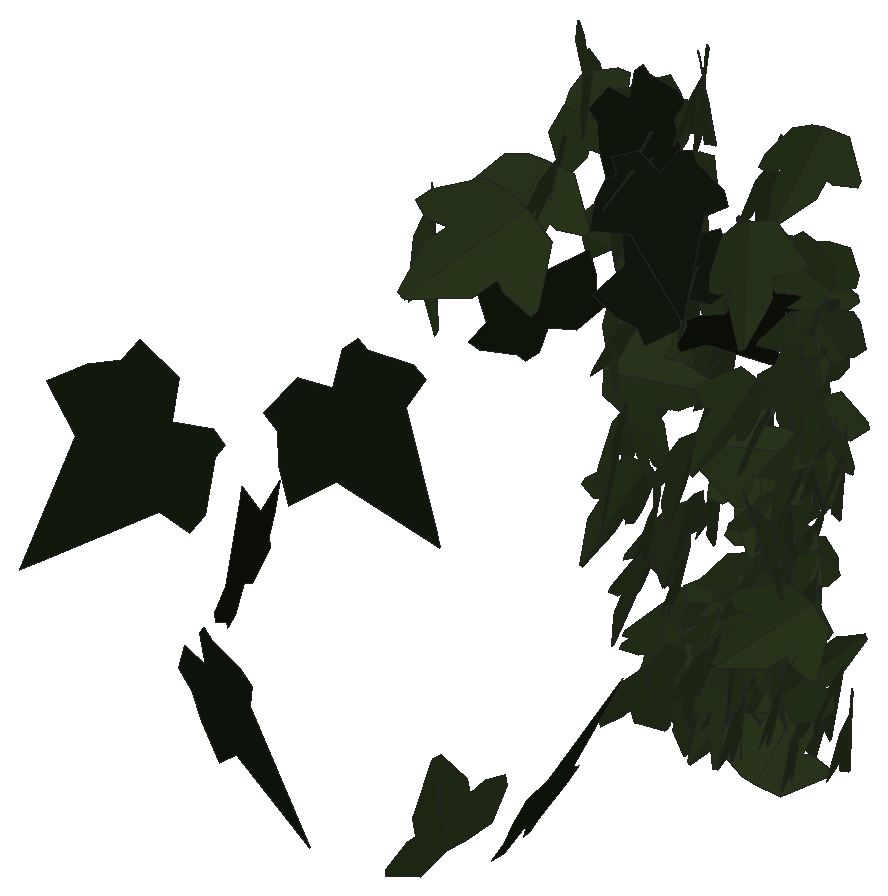
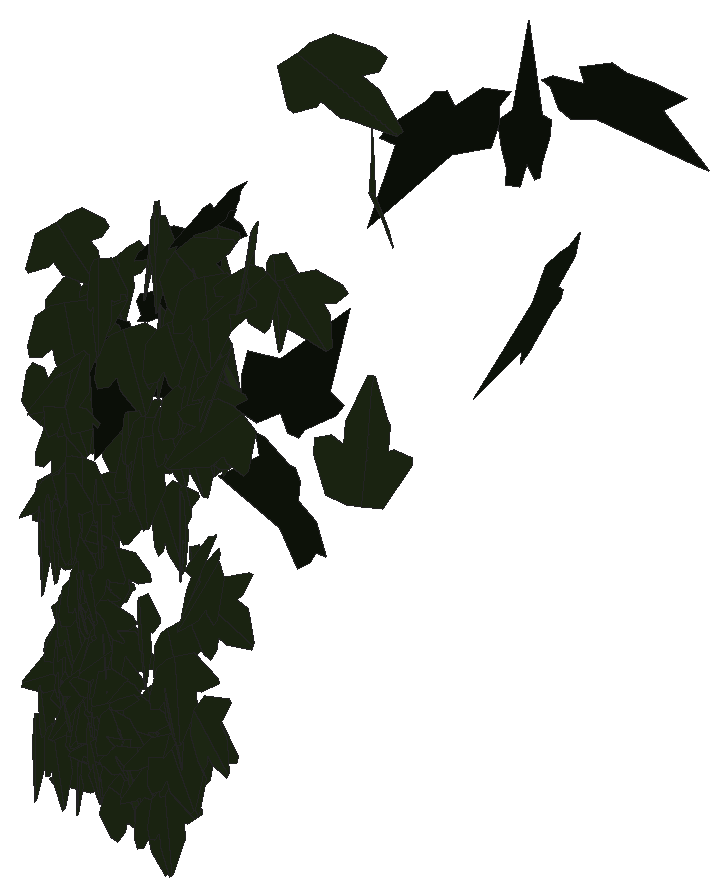
# SketchUp Ruby script. Lengths in inches.
U = 1.inch
M = Sketchup.active_model
def pt(a) = Geom::Point3d.new(a.map { |v| v * U })
def face(e, loops, mat)
  f = e.add_face(loops[0].map { |a| pt(a) })
  loops[1..].each { |l| e.add_face(l.map { |a| pt(a) }).erase! }
  f.material = f.back_material = mat if mat
  f
end
# faces: each face lists its corners as indices into pts; further lists are holes
def faces(e, pts, list, mat = nil) = list.each { |f| face(e, (f[0].is_a?(Array) ? f : [f]).map { |l| l.map { |i| pts[i] } }, mat) }
# xy, xz, yz: faces in a plane at the given z, y or x. An outline is a flat list of corners, or four numbers for a rectangle; further outlines are holes
def ring(l) = l.size == 4 ? [[l[0], l[1]], [l[2], l[1]], [l[2], l[3]], [l[0], l[3]]] : l.each_slice(2).to_a
def flat(e, list, mat, &to3) = list.each { |f| face(e, (f[0].is_a?(Array) ? f : [f]).map { |l| ring(l).map { |u, v| to3.(u, v) } }, mat) }
def xy(e, z, list, mat = nil) = flat(e, list, mat) { |x, y| [x, y, z] }
def xz(e, y, list, mat = nil) = flat(e, list, mat) { |x, z| [x, y, z] }
def yz(e, x, list, mat = nil) = flat(e, list, mat) { |y, z| [x, y, z] }
def lines(e, pts, list) = list.each { |a, b| e.add_line(pt(pts[a]), pt(pts[b])) }
# prism: a flat outline (further loops are holes) pulled along v
def prism(e, loops, v, mat = nil)
  f = face(e, loops, mat); d = Geom::Vector3d.new(v.map { |x| x * U })
  f.pushpull(f.normal.samedirection?(d) ? d.length : -d.length)
end
def box(e, o, s, mat = nil) = prism(e, [[o, [o[0] + s[0], o[1], o[2]], [o[0] + s[0], o[1] + s[1], o[2]], [o[0], o[1] + s[1], o[2]]]], [0, 0, s[2]], mat)
def at(x, y, z, deg = 0) = Geom::Transformation.translation(pt([x, y, z])) * Geom::Transformation.rotation(ORIGIN, Z_AXIS, deg.degrees)
def axes(o, x, y, z) = Geom::Transformation.new([*x, 0, *y, 0, *z, 0, *pt(o).to_a, 1])
def part(name) = M.definitions.add(name)
# library, detail: a bought-in or finely detailed component or shape, given as its bounding box
def library(name, o, s) = part(name).tap { |d| box(d.entities, o, s) }
def detail(e, o, s) = box(e.add_group.entities, o, s)
def put(e, d, t, mat = nil) = e.add_instance(d, t).tap { |i| i.material = mat if mat }
def group(e, t, mat = nil) = e.add_group.tap { |g| g.transformation = t; g.material = mat if mat }.entities
root = M.entities
M.materials.add("efeu1").color = [18, 25, 13]
M.materials.add("efeu2").color = [43, 57, 29]
c1 = part("ivyleaf_10")
p = [[0,0.5,-0.03],[-0.0625,2.02,-0.43],[-0.19,2.01,-0.46],[-0.54,1.05,-0.29],[-0.52,0.625,-0.18],[-0.83,0.76,-0.28],
  [-1.16,0.64,-0.33],[-1.15,0.33,-0.24],[-0.77,-0.39,0.02],[-0.3,-0.51,0.16],[0.04,-0.48,0.23],[-0.02,2.01,-0.4375],
  [-0.06,2.01,-0.43],[0.04,-0.49,0.23],[0.67,-0.49,0.14],[1.38,0.36,-0.2],[1.375,0.51,-0.24],[0.81,0.65,-0.19],
  [0.62,0.59,-0.15],[0.6,1.09,-0.28],[0.5,1.23,-0.31]]
faces(c1.entities,p,[[0,1,2,3,4,5,6,7,8,9,10],[11,12,0,13,14,15,16,17,18,19,20]],"efeu2")
c2 = part("ivyleaf_9")
p = [[1.54,2.16,1.25],[1.36,2.04,1.19],[-0.21,0.99,0.68],[-0.71,1.11,0.82],[-0.85,0.86,0.67],[-0.8,0.17,0.21],
  [-0.9,-0.01,0.1],[-0.67,-0.16,-0.02],[-0.08,-0.08,-0.05],[-0.03,-0.6,-0.4],[0.65,-0.88,-0.66],[0.83,-0.6,-0.49],
  [1.29,-0.42,-0.43],[1.8125,-0.07,-0.26],[1.21,0.44,0.15]]
faces(c2.entities,p,[[0,1,2,3,4,5,6,7,8,9,10,11,12,13,14]],"efeu1")
put(root,c1,axes([498.77,137.96,174.09],[0.169,-0.58916,0.2344],[0.04707,-0.23026,-0.61268],[0.63233,0.17461,-0.01704]))
put(root,c1,axes([498.98,136.23,183.62],[0.22181,-0.25237,-0.641],[-0.15269,0.63865,-0.30428],[0.67176,0.2285,0.14249]))
put(root,c2,axes([499.04,135.21,179.7],[0.2917,0.13697,0.71958],[-0.66782,-0.2685,0.32182],[0.30096,-0.72856,0.01668]))
put(root,c1,axes([498.87,137.54,177.1],[0.09454,-0.25751,-0.64935],[0.04934,0.6561,-0.253],[0.6968,-0.01152,0.10602]))
put(root,c1,axes([498.57,137.53,180.49],[-0.42749,-0.20493,-0.51144],[0.47103,0.19988,-0.47381],[0.28582,-0.6359,0.01589]))
put(root,c1,axes([498.9375,135.04,182.21],[0.61517,0.37241,-0.28496],[-0.24312,-0.14865,-0.71911],[-0.40097,0.66147,-0.00117]))
put(root,c1,axes([498.82,137.39,181.62],[-0.21092,0.66772,0.08289],[-0.00673,0.08477,-0.69999],[-0.67281,-0.21017,-0.01899]))
put(root,c2,axes([499.37,125.42,182.29],[-1.05986,-0.37028,0.11023],[-0.10675,-0.03827,-1.09083],[0.40203,-0.98631,0.00094]))
put(root,c1,axes([498.85,136.36,182.875],[-0.09912,-0.44323,-0.59194],[0.43722,0.44654,-0.40757],[0.5964,-0.40103,0.20041]))
put(root,c1,axes([499.23,135.13,182.51],[0.14096,-0.64935,-0.25041],[-0.0615,0.24288,-0.66443],[0.69324,0.15358,-0.00802]))
put(root,c1,axes([499.22,137.11,176.09],[-0.01704,-0.53595,0.46997],[0.03181,-0.47021,-0.53507],[0.71211,0.00818,0.03515]))
put(root,c1,axes([499.3125,137.19,182.9],[-0.2777,-0.65594,-0.01572],[0.00632,0.01439,-0.71231],[0.6561,-0.27777,0.00021]))
put(root,c1,axes([499.32,138.36,172.28],[-0.0191,-0.63454,-0.11075],[-0.01416,0.11119,-0.63459],[0.64398,-0.01637,-0.01724]))
put(root,c1,axes([499.33,138.07,175.02],[-0.14804,-0.64309,-0.06517],[0.00793,0.06505,-0.65987],[0.64633,-0.14809,-0.00683]))
put(root,c1,axes([499.4,138.1,173.32],[-0.20336,-0.59074,0.1892],[-0.01618,-0.19399,-0.62308],[0.62009,-0.1988,0.04579]))
put(root,c1,axes([499.42,137.98,173.15],[-0.18925,-0.59193,0.19072],[-0.02305,-0.19254,-0.62046],[0.62147,-0.1874,0.03507]))
put(root,c1,axes([499.36,137.16,177.29],[-0.2726,0.54581,0.3087],[-0.11192,0.28886,-0.60955],[-0.61699,-0.29355,-0.02582]))
put(root,c1,axes([499.55,137.32,180.62],[-0.40426,-0.52725,0.21041],[-0.06228,-0.21556,-0.65981],[0.56426,-0.40154,0.07793]))
put(root,c1,axes([499.48,138.05,174.4],[0.29468,-0.58013,-0.09412],[-0.02556,0.09253,-0.6504],[0.58716,0.29518,0.01892]))
put(root,c1,axes([499.55,137.61,178.39],[0.35782,-0.54445,-0.20408],[0.01661,0.2491,-0.63544],[0.5812,0.32808,0.1438]))
put(root,c1,axes([499.62,138.35,172.09],[-0.0688,-0.63941,0.05428],[-0.00276,-0.05429,-0.64309],[0.6417,-0.06879,0.00305]))
put(root,c1,axes([499.53,137.12,181.4],[0.06691,-0.6186,-0.31639],[0.11539,0.32334,-0.60777],[0.68517,0.00596,0.13325]))
put(root,c1,axes([499.49,138.25,173.5],[0.10922,0.6266,0.06189],[-0.00272,0.06328,-0.6359],[-0.62964,0.10842,0.01348]))
put(root,c1,axes([499.68,137.76,175.4],[-0.01368,-0.66531,0.04219],[0.00323,-0.04226,-0.66543],[0.66663,-0.01345,0.00409]))
put(root,c1,axes([499.66,138.28,172.89],[0.05946,0.63243,-0.06084],[-0.05162,-0.0561,-0.63356],[-0.63325,0.06396,0.04593]))
put(root,c1,axes([499.76,136.84,172.98],[-0.1728,-0.62468,-0.28309],[0.06591,0.27546,-0.64808],[0.68266,-0.18473,-0.00908]))
put(root,c1,axes([499.28,132,182.85],[0.35233,-0.21377,0.81136],[0.69929,-0.43521,-0.40561],[0.52365,0.72502,-0.00425]))
put(root,c1,axes([499.97,137.39,181.77],[-0.28369,-0.61148,0.2043],[-0.0022,-0.22229,-0.66836],[0.6447,-0.26982,0.08762]))
put(root,c1,axes([500.13,136.77,183.09],[-0.19807,-0.53893,0.41581],[-0.04923,-0.42058,-0.56856],[0.67891,-0.18773,0.08009]))
put(root,c1,axes([499.69,136.01,179.3],[-0.0556,0.07527,-0.73247],[0.3679,-0.63346,-0.09302],[-0.63783,-0.37193,0.01019]))
put(root,c1,axes([500.17,135.9375,179.78],[0.03815,-0.66931,-0.19407],[-0.03449,0.19231,-0.67002],[0.69603,0.04622,-0.02256]))
put(root,c1,axes([500.01,136.78,179.4],[0.68793,-0.08791,0.00717],[0.00702,-0.00165,-0.69353],[0.08792,0.68797,-0.00075]))
put(root,c1,axes([500.16,137.24,179.88],[0.04716,-0.68441,0.09525],[0.02515,-0.09371,-0.68579],[0.69055,0.05016,0.01848]))
put(root,c1,axes([500.22,136.4,176.35],[0.28246,-0.60836,-0.27966],[-0.08344,0.26918,-0.66983],[0.66434,0.29247,0.03477]))
put(root,c1,axes([500.16,138.0625,176.01],[0.2575,-0.59026,-0.16503],[0.00247,0.18,-0.63996],[0.61289,0.24727,0.07191]))
put(root,c1,axes([500.06,138.26,173.03],[0.54248,0.35695,-0.02191],[-0.01939,-0.01038,-0.64938],[-0.3571,0.54282,0.00199]))
put(root,c1,axes([500.125,138.22,172.53],[-0.5644,0.18765,-0.23674],[0.18425,-0.18371,-0.5849],[-0.23939,-0.58382,0.10796]))
put(root,c1,axes([500.18,136.33,181.53],[0.35706,-0.56386,0.22717],[0.11435,-0.19645,-0.66735],[0.59704,0.37484,-0.00804]))
put(root,c1,axes([500.39,138.42,172.14],[-0.14064,-0.41537,0.46283],[-0.06938,-0.46107,-0.43487],[0.618,-0.14629,0.05651]))
put(root,c1,axes([500.34,138.08,172.55],[0.2401,-0.60033,-0.06449],[-0.0155,0.06325,-0.6465],[0.60359,0.24043,0.00905]))
put(root,c2,axes([499.875,125.91,177.875],[0.81019,-0.64326,-0.32587],[-0.25416,0.20691,-1.02773],[0.72976,0.78622,0.00385]))
put(root,c1,axes([500.51,138.18,173.69],[-0.24109,-0.60692,0.05726],[-0.0345,-0.04789,-0.6529],[0.60864,-0.24313,-0.01433]))
put(root,c1,axes([500.38,138.29,173.18],[-0.53898,-0.33163,-0.13671],[0.16849,-0.01623,-0.62491],[0.31666,-0.55581,0.09981]))
put(root,c1,axes([500.36,136.08,182.83],[0.34824,-0.60547,0.27751],[0.1391,-0.24013,-0.69847],[0.65135,0.37499,0.00079]))
put(root,c1,axes([500.63,137.03,183.71],[0.19784,-0.60344,-0.33031],[-0.06718,0.32511,-0.63417],[0.68464,0.20628,0.03322]))
put(root,c2,axes([500.3125,135.78,183.79],[0.31346,-0.5648,-0.40158],[-0.15249,0.37374,-0.64467],[0.67603,0.34619,0.04079]))
put(root,c1,axes([500.66,137.43,179.03],[-0.16696,-0.66613,-0.05139],[0.00309,0.0522,-0.68667],[0.66811,-0.1667,-0.00966]))
put(root,c1,axes([500.6875,137.09,173.46],[0.11249,-0.65009,-0.01518],[0.00007,0.01541,-0.65975],[0.65027,0.11246,0.00269]))
put(root,c1,axes([500.69,135.44,182.67],[0.13947,-0.69196,0.11409],[0.03515,-0.10928,-0.70577],[0.70043,0.14327,0.0127]))
put(root,c1,axes([500.49,138.38,173.1],[0.40744,0.46805,0.16624],[0.09537,0.1373,-0.6203],[-0.48745,0.41808,0.01759]))
put(root,c1,axes([500.77,136.58,177.46],[0.11316,-0.6648,0.12809],[0.04825,-0.12162,-0.67383],[0.67531,0.12009,0.02668]))
put(root,c1,axes([500.73,136.68,181.33],[-0.10103,0.51742,-0.47375],[-0.06769,-0.48359,-0.51374],[-0.69827,-0.02799,0.11834]))
put(root,c1,axes([500.2,135.86,178.95],[-0.06549,-0.03632,-0.74246],[0.738,0.08607,-0.0693],[0.08901,-0.74036,0.02836]))
put(root,c1,axes([500.71,137.75,172.77],[0.20827,0.56977,-0.20295],[-0.06625,-0.19187,-0.60663],[-0.6012,0.21853,-0.00346]))
put(root,c1,axes([500.81,137.2,179.33],[0.0383,-0.62882,-0.29154],[0.05875,0.29388,-0.62614],[0.69062,0.00987,0.06943]))
put(root,c1,axes([500.74,138.29,173.61],[0.63656,-0.12359,-0.02219],[-0.00957,0.06655,-0.64533],[0.1252,0.63346,0.06347]))
put(root,c1,axes([500.75,138.3,173.8],[0.37049,0.52121,-0.09834],[-0.05575,-0.08102,-0.63946],[-0.52746,0.37465,-0.00148]))
put(root,c1,axes([500.93,137.46,179.51],[0.18136,-0.6149,-0.26073],[-0.03149,0.262,-0.6398],[0.66715,0.17952,0.04068]))
put(root,c1,axes([500.92,138.3125,173.875],[-0.19523,-0.61364,0.05872],[0.03803,-0.07347,-0.64131],[0.61527,-0.19017,0.05828]))
put(root,c1,axes([500.875,136.78,183.79],[0.36981,-0.53867,-0.29794],[0.03431,0.36507,-0.61744],[0.61461,0.30373,0.21374]))
put(root,c1,axes([501.07,138.11,174.87],[0.10388,-0.13127,0.63158],[-0.32258,0.54341,0.166],[-0.55863,-0.33821,0.02159]))
put(root,c1,axes([500.74,138.19,174.2],[0.23417,0.40188,0.4552],[0.08974,0.45962,-0.45195],[-0.60056,0.22539,0.10996]))
put(root,c1,axes([500.99,138.47,173.31],[0.18753,-0.60033,-0.10885],[-0.00545,0.11222,-0.62832],[0.6101,0.18553,0.02785]))
put(root,c1,axes([501.04,137.93,174.91],[-0.44425,-0.48912,-0.03095],[0.04776,-0.00163,-0.65975],[0.48777,-0.44533,0.03641]))
put(root,c1,axes([501.01,137.66,173.72],[-0.13553,0.57627,-0.25871],[-0.07838,-0.2779,-0.57795],[-0.6268,-0.08985,0.12821]))
put(root,c1,axes([501.08,138.06,175.08],[0.29336,-0.54516,-0.20698],[-0.03323,0.21569,-0.6152],[0.58218,0.28702,0.06918]))
put(root,c1,axes([501.11,137.98,173.16],[-0.07059,-0.60616,0.23057],[0.02369,-0.23419,-0.60842],[0.6481,-0.05746,0.04735]))
put(root,c1,axes([501.15,138.02,173.89],[0.00118,-0.65228,0.06383],[-0.00761,-0.06384,-0.65223],[0.65535,0.00043,-0.00769]))
put(root,c1,axes([501.18,138.15,174.23],[0.13806,-0.58633,-0.24066],[-0.01196,0.24385,-0.60096],[0.63369,0.13234,0.04109]))
put(root,c1,axes([501.23,138.06,174.5],[-0.54158,-0.36295,0.01386],[-0.01174,-0.00739,-0.65196],[0.36303,-0.54171,-0.00039]))
put(root,c2,axes([500.97,125.38,180.17],[0.06893,0.48878,0.73074],[-0.23091,-0.67314,0.5072],[0.89509,-0.21129,0.07457]))
put(root,c2,axes([500.83,127.83,182.3],[0.18705,-0.64128,-0.78261],[-0.12387,0.74578,-0.68842],[1.06058,0.2002,0.05762]))
put(root,c1,axes([501.15,136.93,178.86],[0.2891,-0.63741,0.13207],[0.05728,-0.11904,-0.6999],[0.64842,0.29471,0.00294]))
put(root,c1,axes([501.27,137.21,172.73],[0.22485,-0.56327,-0.2545],[-0.02524,0.26223,-0.60266],[0.61758,0.21579,0.06803]))
put(root,c1,axes([501.29,137.78,174.92],[-0.05152,-0.63412,-0.1975],[0.00474,0.19774,-0.63611],[0.66414,-0.0506,-0.01079]))
put(root,c2,axes([501.57,135.39,181.03],[-0.5132,-0.56091,0.15021],[0.1194,0.09425,0.75988],[-0.56826,0.52636,0.02401]))
put(root,c1,axes([501.69,130.78,184.27],[0.70994,0.15773,-0.67825],[-0.68075,-0.16776,-0.70294],[-0.24837,0.91065,-0.01202]))
put(root,c1,axes([501.39,135.95,181.04],[0.26272,-0.53473,-0.38107],[-0.07467,0.38345,-0.58955],[0.65236,0.25924,0.08599]))
put(root,c1,axes([501.17,138.24,174.23],[-0.19526,-0.42206,-0.45564],[0.29367,0.35812,-0.45757],[0.54726,-0.34276,0.08297]))
put(root,c1,axes([501.45,136.92,180.9],[-0.35309,-0.58372,0.16905],[-0.02653,-0.18053,-0.67875],[0.60713,-0.34737,0.06866]))
put(root,c1,axes([501.25,137.78,173.53],[-0.51375,0.36182,-0.17258],[0.13521,-0.10769,-0.6283],[-0.37738,-0.53115,0.00983]))
put(root,c2,axes([501.13,135.44,182.9],[-0.10012,-0.69718,-0.30488],[0.0456,0.30146,-0.70433],[0.75956,-0.10999,0.0021]))
put(root,c1,axes([501.45,138.05,175.56],[0.58538,0.16016,-0.26092],[-0.25499,-0.05654,-0.60678],[-0.16944,0.6384,0.01172]))
put(root,c1,axes([501.26,137.72,176.73],[0.62992,0.22319,0.03324],[0.02744,0.02207,-0.66819],[-0.22398,0.63041,0.01162]))
put(root,c1,axes([501.5,137.91,176.9],[-0.67245,0.05057,0.03675],[-0.03688,-0.00038,-0.67434],[-0.05047,-0.67345,0.00314]))
put(root,c1,axes([501.54,138.03,176.11],[-0.22823,-0.61591,0.08269],[-0.04045,-0.07318,-0.65672],[0.62012,-0.23145,-0.01241]))
put(root,c1,axes([501.57,138.16,175.21],[-0.42629,-0.49666,0.00449],[0.0041,-0.00944,-0.65445],[0.49667,-0.42621,0.00926]))
put(root,c1,axes([501.59,137.48,177.93],[0.14761,-0.59692,-0.29532],[-0.04463,0.29294,-0.61442],[0.66448,0.15227,0.02434]))
put(root,c1,axes([501.77,137.72,174.27],[-0.45768,-0.42721,0.18591],[-0.09159,-0.17301,-0.62307],[0.45681,-0.46271,0.06133]))
put(root,c1,axes([501.68,138.42,173.92],[0.26725,-0.58261,-0.0424],[-0.00935,0.04235,-0.64092],[0.58408,0.26726,0.00914]))
put(root,c1,axes([501.89,137.9,176.61],[0.38287,-0.28571,-0.46144],[-0.31061,0.34773,-0.47303],[0.44507,0.48847,0.06683]))
put(root,c1,axes([501.7,137.97,176.25],[0.08392,-0.63874,-0.13344],[0.01288,0.13613,-0.64354],[0.6524,0.07947,0.02987]))
put(root,c1,axes([501.79,137.5,173.13],[0.2937,-0.5521,-0.18873],[-0.04474,0.18936,-0.62357],[0.58175,0.2933,0.04733]))
put(root,c1,axes([501.8125,137.28,182.45],[0.11966,-0.64549,-0.27399],[-0.02462,0.27391,-0.65606],[0.7008,0.11984,0.02373]))
put(root,c1,axes([501.8,136.62,178.74],[-0.06246,-0.46927,0.50324],[0.04452,-0.50701,-0.46726],[0.68665,-0.00982,0.07607]))
put(root,c1,axes([501.96,137.77,178.3125],[-0.65704,0.08671,0.13728],[-0.14371,-0.04418,-0.65989],[-0.07558,-0.66977,0.0613]))
put(root,c1,axes([501.37,136.88,177.65],[-0.03674,-0.2027,-0.70056],[0.62187,0.35774,-0.13612],[0.38099,-0.60346,0.15463]))
put(root,c1,axes([501.59,137.49,171.8125],[0.54646,0.2779,-0.31031],[0.26065,0.17116,0.61229],[0.32494,-0.60466,0.03071]))
put(root,c1,axes([501.88,138.19,175.62],[0.13611,-0.63707,-0.0697],[-0.01275,0.06854,-0.65144],[0.64074,0.1367,0.00184]))
put(root,c2,axes([501.87,136.21,180.4],[0.37145,0.6692,0.00724],[0.00363,0.00627,-0.76538],[-0.66923,0.37147,-0.00013]))
put(root,c1,axes([501.84,137.81,175.07],[-0.32223,-0.55138,-0.16214],[0.15466,0.09583,-0.63327],[0.55352,-0.34776,0.08256]))
put(root,c1,axes([501.97,138.18,174.77],[0.13015,-0.58817,-0.24812],[-0.01926,0.24949,-0.60153],[0.63807,0.1275,0.03245]))
put(root,c1,axes([501.66,133.71,179.3],[0.46096,-0.46081,0.55084],[0.38094,-0.39799,-0.65172],[0.60881,0.59792,-0.00928]))
put(root,c1,axes([501.98,137.6875,172.38],[0.29319,-0.50509,-0.25376],[-0.01369,0.27943,-0.57201],[0.56508,0.26883,0.1178]))
put(root,c1,axes([501.63,138.04,175.79],[0.1472,-0.15426,0.62818],[0.4829,-0.40242,-0.21198],[0.43036,0.50431,0.023]))
put(root,c1,axes([502.05,138.33,172.73],[0.10827,-0.62752,-0.10166],[-0.0228,0.09922,-0.63677],[0.63529,0.11051,-0.00553]))
put(root,c1,axes([502.07,137.8,177.38],[0.06386,-0.62602,0.23795],[0.05784,-0.23298,-0.62847],[0.66721,0.08011,0.0317]))
put(root,c1,axes([502.34,137.86,177.86],[-0.61139,0.05516,0.27789],[-0.27955,-0.01005,-0.61304],[-0.04604,-0.67151,0.032]))
put(root,c1,axes([502.05,129.09,174.39],[-0.26406,-0.82367,-0.37721],[-0.06081,-0.36111,0.89233],[-0.97008,0.24684,0.04674]))
put(root,c1,axes([502.53,136.93,174.96],[0.44306,0.17571,-0.55178],[-0.52688,-0.16596,-0.47591],[-0.24028,0.68791,0.02613]))
put(root,c1,axes([502.32,136.41,176.8],[-0.57529,0.35322,-0.00911],[0.01364,0.0048,-0.67498],[-0.35308,-0.57534,-0.01122]))
put(root,c1,axes([502.41,137.58,179.9],[-0.08454,-0.66887,0.15832],[-0.01114,-0.15816,-0.67413],[0.68726,-0.08484,0.00854]))
put(root,c1,axes([502.4,137.57,179],[-0.21398,-0.64863,-0.10876],[0.03382,0.10337,-0.68301],[0.65681,-0.21664,-0.00027]))
put(root,c1,axes([502.83,137.03,181.03],[-0.36727,-0.00816,-0.60624],[-0.60627,-0.00048,0.3673],[-0.00464,0.70881,-0.00673]))
put(root,c1,axes([502.41,137.98,177.46],[0.18981,-0.62169,-0.15977],[-0.00047,0.16647,-0.64834],[0.64189,0.18396,0.04677]))
put(root,c1,axes([502.6875,137.74,179.52],[-0.57627,-0.12874,-0.3437],[-0.33861,-0.06035,0.59033],[-0.14159,0.66826,-0.0129]))
put(root,c1,axes([502.32,137.68,180.18],[0.03897,0.6859,-0.01278],[-0.00006,-0.01279,-0.68701],[-0.68602,0.03897,-0.00067]))
put(root,c1,axes([502.49,138.13,173.34],[0.22865,-0.59083,-0.12994],[-0.01194,0.13448,-0.63247],[0.60483,0.22601,0.03663]))
put(root,c1,axes([502.65,137.29,181.22],[-0.51671,-0.45117,0.15095],[-0.05336,-0.16648,-0.68027],[0.47275,-0.51192,0.0882]))
put(root,c1,axes([502.57,138.09,177.2],[0.24214,-0.57742,-0.21843],[-0.00975,0.23103,-0.62152],[0.61728,0.23015,0.07587]))
put(root,c1,axes([502.47,135.98,181.89],[0.16653,0.742,-0.15425],[-0.05277,-0.1462,-0.76022],[-0.75603,0.17364,0.01908]))
put(root,c1,axes([502.68,137.3125,183.14],[0.3391,0.52783,-0.30852],[-0.29508,-0.16768,-0.61122],[-0.53546,0.42668,0.14145]))
put(root,c1,axes([502.48,137.83,178.04],[0.00762,0.67002,-0.10036],[-0.00396,-0.10032,-0.67006],[-0.67749,0.00812,0.00278]))
put(root,c1,axes([502.57,137.16,173.67],[0.06791,-0.15701,0.70428],[-0.11515,0.69597,0.16626],[-0.71232,-0.12747,0.04027]))
put(root,c2,axes([502.625,130.37,174.3],[-0.4676,0.75874,-0.28692],[-0.14773,0.23958,0.90852],[0.85932,0.45406,0.00007]))
put(root,c1,axes([502.69,138.1,172.62],[0.21735,-0.53615,-0.27461],[-0.03295,0.28092,-0.57454],[0.60148,0.20913,0.06776]))
